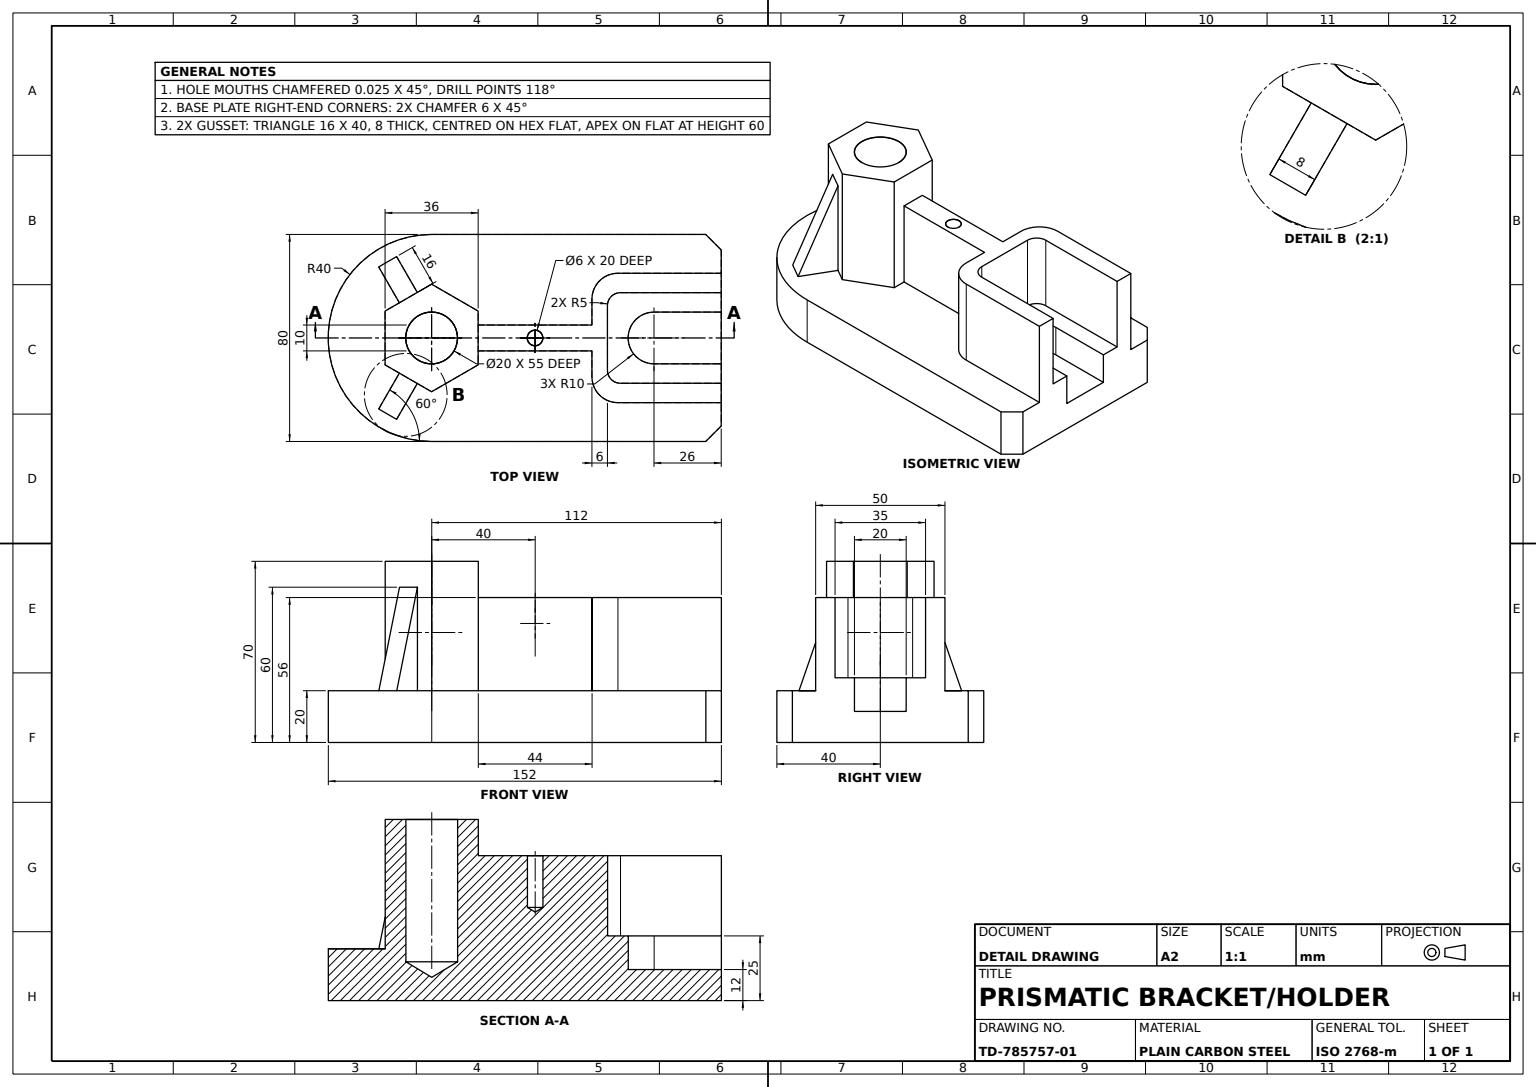
ISO-10303-21;
HEADER;
FILE_DESCRIPTION((''),'2;1');
FILE_NAME('','',(''),(''),'','','');
FILE_SCHEMA(('AUTOMOTIVE_DESIGN'));
ENDSEC;
DATA;
#1=APPLICATION_CONTEXT('');
#2=PRODUCT_CONTEXT('',#1,'mechanical');
#3=PRODUCT('','','',(#2));
#4=PRODUCT_DEFINITION_FORMATION('','',#3);
#5=PRODUCT_DEFINITION_CONTEXT('',#1,'design');
#6=PRODUCT_DEFINITION('','',#4,#5);
#7=PRODUCT_DEFINITION_SHAPE('','',#6);
#8=(LENGTH_UNIT()NAMED_UNIT(*)SI_UNIT(.MILLI.,.METRE.));
#9=(NAMED_UNIT(*)PLANE_ANGLE_UNIT()SI_UNIT($,.RADIAN.));
#10=(NAMED_UNIT(*)SI_UNIT($,.STERADIAN.)SOLID_ANGLE_UNIT());
#11=UNCERTAINTY_MEASURE_WITH_UNIT(LENGTH_MEASURE(1.E-05),#8,'distance_accuracy_value','');
#12=(GEOMETRIC_REPRESENTATION_CONTEXT(3)GLOBAL_UNCERTAINTY_ASSIGNED_CONTEXT((#11))GLOBAL_UNIT_ASSIGNED_CONTEXT((#8,#9,#10))REPRESENTATION_CONTEXT('',''));
#13=CARTESIAN_POINT('',(40.,36.,-3.));
#14=VERTEX_POINT('',#13);
#15=CARTESIAN_POINT('',(40.,55.975,-3.));
#16=VERTEX_POINT('',#15);
#17=CARTESIAN_POINT('',(40.,56.,-3.));
#18=DIRECTION('',(0.,1.,0.));
#19=VECTOR('',#18,1000.);
#20=LINE('',#17,#19);
#21=EDGE_CURVE('',#14,#16,#20,.T.);
#22=ORIENTED_EDGE('',*,*,#21,.T.);
#23=CARTESIAN_POINT('',(40.,55.975,3.));
#24=VERTEX_POINT('',#23);
#25=CARTESIAN_POINT('',(40.,55.975,0.));
#26=DIRECTION('',(0.,0.,1.));
#27=AXIS2_PLACEMENT_3D('',#25,#18,#26);
#28=CIRCLE('',#27,3.);
#29=EDGE_CURVE('',#16,#24,#28,.T.);
#30=ORIENTED_EDGE('',*,*,#29,.T.);
#31=CARTESIAN_POINT('',(40.,36.,3.));
#32=VERTEX_POINT('',#31);
#33=CARTESIAN_POINT('',(40.,56.,3.));
#34=LINE('',#33,#19);
#35=EDGE_CURVE('',#32,#24,#34,.T.);
#36=ORIENTED_EDGE('',*,*,#35,.F.);
#37=CARTESIAN_POINT('',(40.,36.,0.));
#38=AXIS2_PLACEMENT_3D('',#37,#18,#26);
#39=CIRCLE('',#38,3.);
#40=EDGE_CURVE('',#14,#32,#39,.T.);
#41=ORIENTED_EDGE('',*,*,#40,.F.);
#42=EDGE_LOOP('',(#22,#30,#36,#41));
#43=FACE_OUTER_BOUND('',#42,.T.);
#44=CARTESIAN_POINT('',(40.,56.,0.));
#45=AXIS2_PLACEMENT_3D('',#44,#18,#26);
#46=CYLINDRICAL_SURFACE('',#45,3.);
#47=ADVANCED_FACE('',(#43),#46,.F.);
#48=CARTESIAN_POINT('',(62.,56.,15.));
#49=VERTEX_POINT('',#48);
#50=CARTESIAN_POINT('',(62.,20.,15.));
#51=VERTEX_POINT('',#50);
#52=DIRECTION('',(0.,-1.,0.));
#53=VECTOR('',#52,1000.);
#54=LINE('',#48,#53);
#55=EDGE_CURVE('',#49,#51,#54,.T.);
#56=ORIENTED_EDGE('',*,*,#55,.F.);
#57=CARTESIAN_POINT('',(62.,56.,5.));
#58=VERTEX_POINT('',#57);
#59=VECTOR('',#26,1000.);
#60=LINE('',#57,#59);
#61=EDGE_CURVE('',#58,#49,#60,.T.);
#62=ORIENTED_EDGE('',*,*,#61,.F.);
#63=CARTESIAN_POINT('',(62.,20.,5.));
#64=VERTEX_POINT('',#63);
#65=LINE('',#57,#53);
#66=EDGE_CURVE('',#58,#64,#65,.T.);
#67=ORIENTED_EDGE('',*,*,#66,.T.);
#68=LINE('',#63,#59);
#69=EDGE_CURVE('',#64,#51,#68,.T.);
#70=ORIENTED_EDGE('',*,*,#69,.T.);
#71=EDGE_LOOP('',(#56,#62,#67,#70));
#72=FACE_OUTER_BOUND('',#71,.T.);
#73=DIRECTION('',(1.,0.,0.));
#74=DIRECTION('',(0.,0.,-1.));
#75=AXIS2_PLACEMENT_3D('',#57,#73,#74);
#76=PLANE('',#75);
#77=ADVANCED_FACE('',(#72),#76,.F.);
#78=CARTESIAN_POINT('',(68.,56.,12.5));
#79=VERTEX_POINT('',#78);
#80=CARTESIAN_POINT('',(68.,25.,12.5));
#81=VERTEX_POINT('',#80);
#82=LINE('',#78,#53);
#83=EDGE_CURVE('',#79,#81,#82,.T.);
#84=ORIENTED_EDGE('',*,*,#83,.F.);
#85=CARTESIAN_POINT('',(73.,56.,17.5));
#86=VERTEX_POINT('',#85);
#87=CARTESIAN_POINT('',(73.,56.,12.5));
#88=AXIS2_PLACEMENT_3D('',#87,#52,#74);
#89=CIRCLE('',#88,5.);
#90=EDGE_CURVE('',#86,#79,#89,.T.);
#91=ORIENTED_EDGE('',*,*,#90,.F.);
#92=CARTESIAN_POINT('',(73.,25.,17.5));
#93=VERTEX_POINT('',#92);
#94=LINE('',#85,#53);
#95=EDGE_CURVE('',#86,#93,#94,.T.);
#96=ORIENTED_EDGE('',*,*,#95,.T.);
#97=CARTESIAN_POINT('',(73.,25.,12.5));
#98=AXIS2_PLACEMENT_3D('',#97,#18,#26);
#99=CIRCLE('',#98,5.);
#100=EDGE_CURVE('',#81,#93,#99,.T.);
#101=ORIENTED_EDGE('',*,*,#100,.F.);
#102=EDGE_LOOP('',(#84,#91,#96,#101));
#103=FACE_OUTER_BOUND('',#102,.T.);
#104=CYLINDRICAL_SURFACE('',#88,5.);
#105=ADVANCED_FACE('',(#103),#104,.F.);
#106=CARTESIAN_POINT('',(68.,25.,-12.5));
#107=VERTEX_POINT('',#106);
#108=LINE('',#106,#59);
#109=EDGE_CURVE('',#107,#81,#108,.T.);
#110=ORIENTED_EDGE('',*,*,#109,.F.);
#111=CARTESIAN_POINT('',(68.,56.,-12.5));
#112=VERTEX_POINT('',#111);
#113=LINE('',#111,#53);
#114=EDGE_CURVE('',#112,#107,#113,.T.);
#115=ORIENTED_EDGE('',*,*,#114,.F.);
#116=VECTOR('',#74,1000.);
#117=LINE('',#78,#116);
#118=EDGE_CURVE('',#79,#112,#117,.T.);
#119=ORIENTED_EDGE('',*,*,#118,.F.);
#120=ORIENTED_EDGE('',*,*,#83,.T.);
#121=EDGE_LOOP('',(#110,#115,#119,#120));
#122=FACE_OUTER_BOUND('',#121,.T.);
#123=DIRECTION('',(-1.,0.,0.));
#124=AXIS2_PLACEMENT_3D('',#78,#123,#26);
#125=PLANE('',#124);
#126=ADVANCED_FACE('',(#122),#125,.F.);
#127=CARTESIAN_POINT('',(-12.464102,60.,-13.588457));
#128=VERTEX_POINT('',#127);
#129=CARTESIAN_POINT('',(-5.535898,60.,-17.588457));
#130=VERTEX_POINT('',#129);
#131=DIRECTION('',(0.866025404,0.,-0.5));
#132=VECTOR('',#131,1000.);
#133=LINE('',#129,#132);
#134=EDGE_CURVE('',#128,#130,#133,.T.);
#135=ORIENTED_EDGE('',*,*,#134,.T.);
#136=CARTESIAN_POINT('',(-13.535898,20.,-31.444864));
#137=VERTEX_POINT('',#136);
#138=CARTESIAN_POINT('',(-6.639347,54.482759,-19.499686));
#139=DIRECTION('',(0.185695338,0.928476691,0.32163376));
#140=VECTOR('',#139,1000.);
#141=LINE('',#138,#140);
#142=EDGE_CURVE('',#137,#130,#141,.T.);
#143=ORIENTED_EDGE('',*,*,#142,.F.);
#144=CARTESIAN_POINT('',(-20.464102,20.,-27.444864));
#145=VERTEX_POINT('',#144);
#146=DIRECTION('',(-0.866025404,0.,0.5));
#147=VECTOR('',#146,1000.);
#148=LINE('',#136,#147);
#149=EDGE_CURVE('',#137,#145,#148,.T.);
#150=ORIENTED_EDGE('',*,*,#149,.T.);
#151=LINE('',#127,#140);
#152=EDGE_CURVE('',#145,#128,#151,.T.);
#153=ORIENTED_EDGE('',*,*,#152,.T.);
#154=EDGE_LOOP('',(#135,#143,#150,#153));
#155=FACE_OUTER_BOUND('',#154,.T.);
#156=CARTESIAN_POINT('',(-221.915759,60.,107.338513));
#157=DIRECTION('',(0.464238345,-0.371390676,0.804084401));
#158=AXIS2_PLACEMENT_3D('',#156,#157,#131);
#159=PLANE('',#158);
#160=ADVANCED_FACE('',(#155),#159,.F.);
#161=CARTESIAN_POINT('',(106.,20.,-40.));
#162=VERTEX_POINT('',#161);
#163=CARTESIAN_POINT('',(106.,0.,-40.));
#164=VERTEX_POINT('',#163);
#165=LINE('',#161,#53);
#166=EDGE_CURVE('',#162,#164,#165,.T.);
#167=ORIENTED_EDGE('',*,*,#166,.F.);
#168=CARTESIAN_POINT('',(112.,20.,-34.));
#169=VERTEX_POINT('',#168);
#170=DIRECTION('',(-0.707106781,0.,-0.707106781));
#171=VECTOR('',#170,1000.);
#172=LINE('',#161,#171);
#173=EDGE_CURVE('',#169,#162,#172,.T.);
#174=ORIENTED_EDGE('',*,*,#173,.F.);
#175=CARTESIAN_POINT('',(112.,0.,-34.));
#176=VERTEX_POINT('',#175);
#177=LINE('',#168,#53);
#178=EDGE_CURVE('',#169,#176,#177,.T.);
#179=ORIENTED_EDGE('',*,*,#178,.T.);
#180=LINE('',#163,#171);
#181=EDGE_CURVE('',#176,#164,#180,.T.);
#182=ORIENTED_EDGE('',*,*,#181,.T.);
#183=EDGE_LOOP('',(#167,#174,#179,#182));
#184=FACE_OUTER_BOUND('',#183,.T.);
#185=DIRECTION('',(-0.707106781,0.,0.707106781));
#186=DIRECTION('',(0.707106781,0.,0.707106781));
#187=AXIS2_PLACEMENT_3D('',#161,#185,#186);
#188=PLANE('',#187);
#189=ADVANCED_FACE('',(#184),#188,.F.);
#190=CARTESIAN_POINT('',(-13.535898,20.,31.444864));
#191=VERTEX_POINT('',#190);
#192=CARTESIAN_POINT('',(-5.535898,20.,17.588457));
#193=VERTEX_POINT('',#192);
#194=DIRECTION('',(0.5,0.,-0.866025404));
#195=VECTOR('',#194,1000.);
#196=LINE('',#190,#195);
#197=EDGE_CURVE('',#191,#193,#196,.T.);
#198=ORIENTED_EDGE('',*,*,#197,.F.);
#199=CARTESIAN_POINT('',(-20.464102,20.,27.444864));
#200=VERTEX_POINT('',#199);
#201=DIRECTION('',(0.866025404,0.,0.5));
#202=VECTOR('',#201,1000.);
#203=LINE('',#199,#202);
#204=EDGE_CURVE('',#200,#191,#203,.T.);
#205=ORIENTED_EDGE('',*,*,#204,.F.);
#206=CARTESIAN_POINT('',(-12.464102,20.,13.588457));
#207=VERTEX_POINT('',#206);
#208=LINE('',#199,#195);
#209=EDGE_CURVE('',#200,#207,#208,.T.);
#210=ORIENTED_EDGE('',*,*,#209,.T.);
#211=CARTESIAN_POINT('',(-18.,20.,10.392305));
#212=VERTEX_POINT('',#211);
#213=LINE('',#211,#202);
#214=EDGE_CURVE('',#212,#207,#213,.T.);
#215=ORIENTED_EDGE('',*,*,#214,.F.);
#216=CARTESIAN_POINT('',(-18.,20.,-10.392305));
#217=VERTEX_POINT('',#216);
#218=LINE('',#216,#59);
#219=EDGE_CURVE('',#217,#212,#218,.T.);
#220=ORIENTED_EDGE('',*,*,#219,.F.);
#221=CARTESIAN_POINT('',(-12.464102,20.,-13.588457));
#222=VERTEX_POINT('',#221);
#223=CARTESIAN_POINT('',(0.,20.,-20.78461));
#224=LINE('',#223,#147);
#225=EDGE_CURVE('',#222,#217,#224,.T.);
#226=ORIENTED_EDGE('',*,*,#225,.F.);
#227=DIRECTION('',(0.5,0.,0.866025404));
#228=VECTOR('',#227,1000.);
#229=LINE('',#144,#228);
#230=EDGE_CURVE('',#145,#222,#229,.T.);
#231=ORIENTED_EDGE('',*,*,#230,.F.);
#232=ORIENTED_EDGE('',*,*,#149,.F.);
#233=CARTESIAN_POINT('',(-5.535898,20.,-17.588457));
#234=VERTEX_POINT('',#233);
#235=LINE('',#136,#228);
#236=EDGE_CURVE('',#137,#234,#235,.T.);
#237=ORIENTED_EDGE('',*,*,#236,.T.);
#238=VERTEX_POINT('',#223);
#239=EDGE_CURVE('',#238,#234,#224,.T.);
#240=ORIENTED_EDGE('',*,*,#239,.F.);
#241=CARTESIAN_POINT('',(18.,20.,-10.392305));
#242=VERTEX_POINT('',#241);
#243=DIRECTION('',(-0.866025404,0.,-0.5));
#244=VECTOR('',#243,1000.);
#245=LINE('',#241,#244);
#246=EDGE_CURVE('',#242,#238,#245,.T.);
#247=ORIENTED_EDGE('',*,*,#246,.F.);
#248=CARTESIAN_POINT('',(18.,20.,-5.));
#249=VERTEX_POINT('',#248);
#250=CARTESIAN_POINT('',(18.,20.,10.392305));
#251=LINE('',#250,#116);
#252=EDGE_CURVE('',#249,#242,#251,.T.);
#253=ORIENTED_EDGE('',*,*,#252,.F.);
#254=CARTESIAN_POINT('',(62.,20.,-5.));
#255=VERTEX_POINT('',#254);
#256=VECTOR('',#123,1000.);
#257=LINE('',#248,#256);
#258=EDGE_CURVE('',#255,#249,#257,.T.);
#259=ORIENTED_EDGE('',*,*,#258,.F.);
#260=CARTESIAN_POINT('',(62.,20.,-15.));
#261=VERTEX_POINT('',#260);
#262=LINE('',#260,#59);
#263=EDGE_CURVE('',#261,#255,#262,.T.);
#264=ORIENTED_EDGE('',*,*,#263,.F.);
#265=CARTESIAN_POINT('',(72.,20.,-25.));
#266=VERTEX_POINT('',#265);
#267=CARTESIAN_POINT('',(72.,20.,-15.));
#268=AXIS2_PLACEMENT_3D('',#267,#18,#26);
#269=CIRCLE('',#268,10.);
#270=EDGE_CURVE('',#266,#261,#269,.T.);
#271=ORIENTED_EDGE('',*,*,#270,.F.);
#272=CARTESIAN_POINT('',(112.,20.,-25.));
#273=VERTEX_POINT('',#272);
#274=LINE('',#272,#256);
#275=EDGE_CURVE('',#273,#266,#274,.T.);
#276=ORIENTED_EDGE('',*,*,#275,.F.);
#277=LINE('',#168,#116);
#278=EDGE_CURVE('',#273,#169,#277,.T.);
#279=ORIENTED_EDGE('',*,*,#278,.T.);
#280=ORIENTED_EDGE('',*,*,#173,.T.);
#281=CARTESIAN_POINT('',(0.,20.,-40.));
#282=VERTEX_POINT('',#281);
#283=LINE('',#281,#256);
#284=EDGE_CURVE('',#162,#282,#283,.T.);
#285=ORIENTED_EDGE('',*,*,#284,.T.);
#286=CARTESIAN_POINT('',(0.,20.,40.));
#287=VERTEX_POINT('',#286);
#288=CARTESIAN_POINT('',(0.,20.,0.));
#289=AXIS2_PLACEMENT_3D('',#288,#18,#26);
#290=CIRCLE('',#289,40.);
#291=EDGE_CURVE('',#282,#287,#290,.T.);
#292=ORIENTED_EDGE('',*,*,#291,.T.);
#293=CARTESIAN_POINT('',(106.,20.,40.));
#294=VERTEX_POINT('',#293);
#295=VECTOR('',#73,1000.);
#296=LINE('',#293,#295);
#297=EDGE_CURVE('',#287,#294,#296,.T.);
#298=ORIENTED_EDGE('',*,*,#297,.T.);
#299=CARTESIAN_POINT('',(112.,20.,34.));
#300=VERTEX_POINT('',#299);
#301=DIRECTION('',(0.707106781,0.,-0.707106781));
#302=VECTOR('',#301,1000.);
#303=LINE('',#299,#302);
#304=EDGE_CURVE('',#294,#300,#303,.T.);
#305=ORIENTED_EDGE('',*,*,#304,.T.);
#306=CARTESIAN_POINT('',(112.,20.,25.));
#307=VERTEX_POINT('',#306);
#308=EDGE_CURVE('',#300,#307,#277,.T.);
#309=ORIENTED_EDGE('',*,*,#308,.T.);
#310=CARTESIAN_POINT('',(72.,20.,25.));
#311=VERTEX_POINT('',#310);
#312=LINE('',#310,#295);
#313=EDGE_CURVE('',#311,#307,#312,.T.);
#314=ORIENTED_EDGE('',*,*,#313,.F.);
#315=CARTESIAN_POINT('',(72.,20.,15.));
#316=AXIS2_PLACEMENT_3D('',#315,#18,#26);
#317=CIRCLE('',#316,10.);
#318=EDGE_CURVE('',#51,#311,#317,.T.);
#319=ORIENTED_EDGE('',*,*,#318,.F.);
#320=ORIENTED_EDGE('',*,*,#69,.F.);
#321=CARTESIAN_POINT('',(18.,20.,5.));
#322=VERTEX_POINT('',#321);
#323=LINE('',#321,#295);
#324=EDGE_CURVE('',#322,#64,#323,.T.);
#325=ORIENTED_EDGE('',*,*,#324,.F.);
#326=VERTEX_POINT('',#250);
#327=EDGE_CURVE('',#326,#322,#251,.T.);
#328=ORIENTED_EDGE('',*,*,#327,.F.);
#329=CARTESIAN_POINT('',(0.,20.,20.78461));
#330=VERTEX_POINT('',#329);
#331=LINE('',#329,#132);
#332=EDGE_CURVE('',#330,#326,#331,.T.);
#333=ORIENTED_EDGE('',*,*,#332,.F.);
#334=EDGE_CURVE('',#193,#330,#213,.T.);
#335=ORIENTED_EDGE('',*,*,#334,.F.);
#336=EDGE_LOOP('',(#198,#205,#210,#215,#220,#226,#231,#232,#237,#240,#247,#253,#259,#264,#271,#276,#279,#280,#285,#292,#298,#305,#309,#314,#319,#320,#325,#328,#333,#335));
#337=FACE_OUTER_BOUND('',#336,.T.);
#338=PLANE('',#289);
#339=ADVANCED_FACE('',(#337),#338,.T.);
#340=CARTESIAN_POINT('',(112.,25.,10.));
#341=VERTEX_POINT('',#340);
#342=CARTESIAN_POINT('',(86.,25.,10.));
#343=VERTEX_POINT('',#342);
#344=LINE('',#340,#256);
#345=EDGE_CURVE('',#341,#343,#344,.T.);
#346=ORIENTED_EDGE('',*,*,#345,.T.);
#347=CARTESIAN_POINT('',(86.,25.,-10.));
#348=VERTEX_POINT('',#347);
#349=CARTESIAN_POINT('',(86.,25.,0.));
#350=AXIS2_PLACEMENT_3D('',#349,#52,#74);
#351=CIRCLE('',#350,10.);
#352=EDGE_CURVE('',#343,#348,#351,.T.);
#353=ORIENTED_EDGE('',*,*,#352,.T.);
#354=CARTESIAN_POINT('',(112.,25.,-10.));
#355=VERTEX_POINT('',#354);
#356=LINE('',#347,#295);
#357=EDGE_CURVE('',#348,#355,#356,.T.);
#358=ORIENTED_EDGE('',*,*,#357,.T.);
#359=CARTESIAN_POINT('',(112.,25.,-17.5));
#360=VERTEX_POINT('',#359);
#361=LINE('',#354,#116);
#362=EDGE_CURVE('',#355,#360,#361,.T.);
#363=ORIENTED_EDGE('',*,*,#362,.T.);
#364=CARTESIAN_POINT('',(73.,25.,-17.5));
#365=VERTEX_POINT('',#364);
#366=LINE('',#359,#256);
#367=EDGE_CURVE('',#360,#365,#366,.T.);
#368=ORIENTED_EDGE('',*,*,#367,.T.);
#369=CARTESIAN_POINT('',(73.,25.,-12.5));
#370=AXIS2_PLACEMENT_3D('',#369,#18,#26);
#371=CIRCLE('',#370,5.);
#372=EDGE_CURVE('',#365,#107,#371,.T.);
#373=ORIENTED_EDGE('',*,*,#372,.T.);
#374=ORIENTED_EDGE('',*,*,#109,.T.);
#375=ORIENTED_EDGE('',*,*,#100,.T.);
#376=CARTESIAN_POINT('',(112.,25.,17.5));
#377=VERTEX_POINT('',#376);
#378=LINE('',#92,#295);
#379=EDGE_CURVE('',#93,#377,#378,.T.);
#380=ORIENTED_EDGE('',*,*,#379,.T.);
#381=LINE('',#376,#116);
#382=EDGE_CURVE('',#377,#341,#381,.T.);
#383=ORIENTED_EDGE('',*,*,#382,.T.);
#384=EDGE_LOOP('',(#346,#353,#358,#363,#368,#373,#374,#375,#380,#383));
#385=FACE_OUTER_BOUND('',#384,.T.);
#386=PLANE('',#370);
#387=ADVANCED_FACE('',(#385),#386,.T.);
#388=ORIENTED_EDGE('',*,*,#313,.T.);
#389=CARTESIAN_POINT('',(112.,56.,25.));
#390=VERTEX_POINT('',#389);
#391=LINE('',#389,#53);
#392=EDGE_CURVE('',#390,#307,#391,.T.);
#393=ORIENTED_EDGE('',*,*,#392,.F.);
#394=CARTESIAN_POINT('',(72.,56.,25.));
#395=VERTEX_POINT('',#394);
#396=LINE('',#394,#295);
#397=EDGE_CURVE('',#395,#390,#396,.T.);
#398=ORIENTED_EDGE('',*,*,#397,.F.);
#399=LINE('',#394,#53);
#400=EDGE_CURVE('',#395,#311,#399,.T.);
#401=ORIENTED_EDGE('',*,*,#400,.T.);
#402=EDGE_LOOP('',(#388,#393,#398,#401));
#403=FACE_OUTER_BOUND('',#402,.T.);
#404=AXIS2_PLACEMENT_3D('',#394,#74,#123);
#405=PLANE('',#404);
#406=ADVANCED_FACE('',(#403),#405,.F.);
#407=EDGE_CURVE('',#24,#16,#28,.T.);
#408=ORIENTED_EDGE('',*,*,#407,.F.);
#409=CARTESIAN_POINT('',(40.,56.,3.025));
#410=VERTEX_POINT('',#409);
#411=DIRECTION('',(0.,0.707106781,0.707106781));
#412=VECTOR('',#411,1000.);
#413=LINE('',#409,#412);
#414=EDGE_CURVE('',#24,#410,#413,.T.);
#415=ORIENTED_EDGE('',*,*,#414,.T.);
#416=CARTESIAN_POINT('',(40.,56.,-3.025));
#417=VERTEX_POINT('',#416);
#418=CIRCLE('',#45,3.025);
#419=EDGE_CURVE('',#410,#417,#418,.T.);
#420=ORIENTED_EDGE('',*,*,#419,.T.);
#421=DIRECTION('',(0.,0.707106781,-0.707106781));
#422=VECTOR('',#421,1000.);
#423=LINE('',#416,#422);
#424=EDGE_CURVE('',#16,#417,#423,.T.);
#425=ORIENTED_EDGE('',*,*,#424,.F.);
#426=EDGE_LOOP('',(#408,#415,#420,#425));
#427=FACE_OUTER_BOUND('',#426,.T.);
#428=CONICAL_SURFACE('',#45,3.025,0.785398163);
#429=ADVANCED_FACE('',(#427),#428,.F.);
#430=CARTESIAN_POINT('',(0.,0.,-40.));
#431=VERTEX_POINT('',#430);
#432=LINE('',#430,#256);
#433=EDGE_CURVE('',#164,#431,#432,.T.);
#434=ORIENTED_EDGE('',*,*,#433,.T.);
#435=LINE('',#281,#53);
#436=EDGE_CURVE('',#282,#431,#435,.T.);
#437=ORIENTED_EDGE('',*,*,#436,.F.);
#438=ORIENTED_EDGE('',*,*,#284,.F.);
#439=ORIENTED_EDGE('',*,*,#166,.T.);
#440=EDGE_LOOP('',(#434,#437,#438,#439));
#441=FACE_OUTER_BOUND('',#440,.T.);
#442=AXIS2_PLACEMENT_3D('',#281,#26,#73);
#443=PLANE('',#442);
#444=ADVANCED_FACE('',(#441),#443,.F.);
#445=CARTESIAN_POINT('',(0.,8.991394,0.));
#446=VERTEX_POINT('',#445);
#447=CARTESIAN_POINT('',(0.,15.,10.));
#448=VERTEX_POINT('',#447);
#449=DIRECTION('',(0.,0.515038075,0.857167301));
#450=VECTOR('',#449,1000.);
#451=LINE('',#447,#450);
#452=EDGE_CURVE('',#446,#448,#451,.T.);
#453=ORIENTED_EDGE('',*,*,#452,.T.);
#454=CARTESIAN_POINT('',(0.,15.,-10.));
#455=VERTEX_POINT('',#454);
#456=CARTESIAN_POINT('',(0.,15.,0.));
#457=AXIS2_PLACEMENT_3D('',#456,#18,#26);
#458=CIRCLE('',#457,10.);
#459=EDGE_CURVE('',#448,#455,#458,.T.);
#460=ORIENTED_EDGE('',*,*,#459,.T.);
#461=DIRECTION('',(0.,0.515038075,-0.857167301));
#462=VECTOR('',#461,1000.);
#463=LINE('',#454,#462);
#464=EDGE_CURVE('',#446,#455,#463,.T.);
#465=ORIENTED_EDGE('',*,*,#464,.F.);
#466=EDGE_LOOP('',(#453,#460,#465));
#467=FACE_OUTER_BOUND('',#466,.T.);
#468=CONICAL_SURFACE('',#457,10.,1.029744259);
#469=ADVANCED_FACE('',(#467),#468,.F.);
#470=CARTESIAN_POINT('',(106.,0.,40.));
#471=VERTEX_POINT('',#470);
#472=CARTESIAN_POINT('',(112.,0.,34.));
#473=VERTEX_POINT('',#472);
#474=LINE('',#472,#302);
#475=EDGE_CURVE('',#471,#473,#474,.T.);
#476=ORIENTED_EDGE('',*,*,#475,.T.);
#477=LINE('',#299,#53);
#478=EDGE_CURVE('',#300,#473,#477,.T.);
#479=ORIENTED_EDGE('',*,*,#478,.F.);
#480=ORIENTED_EDGE('',*,*,#304,.F.);
#481=LINE('',#293,#53);
#482=EDGE_CURVE('',#294,#471,#481,.T.);
#483=ORIENTED_EDGE('',*,*,#482,.T.);
#484=EDGE_LOOP('',(#476,#479,#480,#483));
#485=FACE_OUTER_BOUND('',#484,.T.);
#486=AXIS2_PLACEMENT_3D('',#299,#170,#185);
#487=PLANE('',#486);
#488=ADVANCED_FACE('',(#485),#487,.F.);
#489=CARTESIAN_POINT('',(0.,69.975,10.));
#490=VERTEX_POINT('',#489);
#491=CARTESIAN_POINT('',(0.,70.,10.025));
#492=VERTEX_POINT('',#491);
#493=LINE('',#491,#412);
#494=EDGE_CURVE('',#490,#492,#493,.T.);
#495=ORIENTED_EDGE('',*,*,#494,.T.);
#496=CARTESIAN_POINT('',(0.,70.,-10.025));
#497=VERTEX_POINT('',#496);
#498=CARTESIAN_POINT('',(0.,70.,0.));
#499=AXIS2_PLACEMENT_3D('',#498,#18,#26);
#500=CIRCLE('',#499,10.025);
#501=EDGE_CURVE('',#492,#497,#500,.T.);
#502=ORIENTED_EDGE('',*,*,#501,.T.);
#503=CARTESIAN_POINT('',(0.,69.975,-10.));
#504=VERTEX_POINT('',#503);
#505=LINE('',#496,#422);
#506=EDGE_CURVE('',#504,#497,#505,.T.);
#507=ORIENTED_EDGE('',*,*,#506,.F.);
#508=CARTESIAN_POINT('',(0.,69.975,0.));
#509=AXIS2_PLACEMENT_3D('',#508,#18,#26);
#510=CIRCLE('',#509,10.);
#511=EDGE_CURVE('',#490,#504,#510,.T.);
#512=ORIENTED_EDGE('',*,*,#511,.F.);
#513=EDGE_LOOP('',(#495,#502,#507,#512));
#514=FACE_OUTER_BOUND('',#513,.T.);
#515=CONICAL_SURFACE('',#499,10.025,0.785398163);
#516=ADVANCED_FACE('',(#514),#515,.F.);
#517=ORIENTED_EDGE('',*,*,#414,.F.);
#518=ORIENTED_EDGE('',*,*,#29,.F.);
#519=ORIENTED_EDGE('',*,*,#424,.T.);
#520=EDGE_CURVE('',#417,#410,#418,.T.);
#521=ORIENTED_EDGE('',*,*,#520,.T.);
#522=EDGE_LOOP('',(#517,#518,#519,#521));
#523=FACE_OUTER_BOUND('',#522,.T.);
#524=ADVANCED_FACE('',(#523),#428,.F.);
#525=ORIENTED_EDGE('',*,*,#452,.F.);
#526=ORIENTED_EDGE('',*,*,#464,.T.);
#527=EDGE_CURVE('',#455,#448,#458,.T.);
#528=ORIENTED_EDGE('',*,*,#527,.T.);
#529=EDGE_LOOP('',(#525,#526,#528));
#530=FACE_OUTER_BOUND('',#529,.T.);
#531=ADVANCED_FACE('',(#530),#468,.F.);
#532=ORIENTED_EDGE('',*,*,#197,.T.);
#533=CARTESIAN_POINT('',(-5.535898,60.,17.588457));
#534=VERTEX_POINT('',#533);
#535=LINE('',#533,#19);
#536=EDGE_CURVE('',#193,#534,#535,.T.);
#537=ORIENTED_EDGE('',*,*,#536,.T.);
#538=DIRECTION('',(0.185695338,0.928476691,-0.32163376));
#539=VECTOR('',#538,1000.);
#540=LINE('',#533,#539);
#541=EDGE_CURVE('',#191,#534,#540,.T.);
#542=ORIENTED_EDGE('',*,*,#541,.F.);
#543=EDGE_LOOP('',(#532,#537,#542));
#544=FACE_OUTER_BOUND('',#543,.T.);
#545=CARTESIAN_POINT('',(-13.535898,60.,31.444864));
#546=DIRECTION('',(-0.5,0.,0.866025404));
#547=AXIS2_PLACEMENT_3D('',#545,#243,#546);
#548=PLANE('',#547);
#549=ADVANCED_FACE('',(#544),#548,.F.);
#550=ORIENTED_EDGE('',*,*,#152,.F.);
#551=ORIENTED_EDGE('',*,*,#230,.T.);
#552=LINE('',#127,#19);
#553=EDGE_CURVE('',#222,#128,#552,.T.);
#554=ORIENTED_EDGE('',*,*,#553,.T.);
#555=EDGE_LOOP('',(#550,#551,#554));
#556=FACE_OUTER_BOUND('',#555,.T.);
#557=CARTESIAN_POINT('',(-20.464102,60.,-27.444864));
#558=DIRECTION('',(-0.5,0.,-0.866025404));
#559=AXIS2_PLACEMENT_3D('',#557,#131,#558);
#560=PLANE('',#559);
#561=ADVANCED_FACE('',(#556),#560,.F.);
#562=ORIENTED_EDGE('',*,*,#291,.F.);
#563=ORIENTED_EDGE('',*,*,#436,.T.);
#564=CARTESIAN_POINT('',(0.,0.,40.));
#565=VERTEX_POINT('',#564);
#566=CARTESIAN_POINT('',(0.,0.,0.));
#567=AXIS2_PLACEMENT_3D('',#566,#18,#26);
#568=CIRCLE('',#567,40.);
#569=EDGE_CURVE('',#431,#565,#568,.T.);
#570=ORIENTED_EDGE('',*,*,#569,.T.);
#571=LINE('',#286,#53);
#572=EDGE_CURVE('',#287,#565,#571,.T.);
#573=ORIENTED_EDGE('',*,*,#572,.F.);
#574=EDGE_LOOP('',(#562,#563,#570,#573));
#575=FACE_OUTER_BOUND('',#574,.T.);
#576=AXIS2_PLACEMENT_3D('',#288,#52,#74);
#577=CYLINDRICAL_SURFACE('',#576,40.);
#578=ADVANCED_FACE('',(#575),#577,.T.);
#579=CARTESIAN_POINT('',(112.,56.,-25.));
#580=VERTEX_POINT('',#579);
#581=CARTESIAN_POINT('',(72.,56.,-25.));
#582=VERTEX_POINT('',#581);
#583=LINE('',#579,#256);
#584=EDGE_CURVE('',#580,#582,#583,.T.);
#585=ORIENTED_EDGE('',*,*,#584,.F.);
#586=LINE('',#579,#53);
#587=EDGE_CURVE('',#580,#273,#586,.T.);
#588=ORIENTED_EDGE('',*,*,#587,.T.);
#589=ORIENTED_EDGE('',*,*,#275,.T.);
#590=LINE('',#581,#53);
#591=EDGE_CURVE('',#582,#266,#590,.T.);
#592=ORIENTED_EDGE('',*,*,#591,.F.);
#593=EDGE_LOOP('',(#585,#588,#589,#592));
#594=FACE_OUTER_BOUND('',#593,.T.);
#595=AXIS2_PLACEMENT_3D('',#579,#26,#73);
#596=PLANE('',#595);
#597=ADVANCED_FACE('',(#594),#596,.F.);
#598=CARTESIAN_POINT('',(0.,70.,-10.));
#599=LINE('',#598,#19);
#600=EDGE_CURVE('',#455,#504,#599,.T.);
#601=ORIENTED_EDGE('',*,*,#600,.T.);
#602=EDGE_CURVE('',#504,#490,#510,.T.);
#603=ORIENTED_EDGE('',*,*,#602,.T.);
#604=CARTESIAN_POINT('',(0.,70.,10.));
#605=LINE('',#604,#19);
#606=EDGE_CURVE('',#448,#490,#605,.T.);
#607=ORIENTED_EDGE('',*,*,#606,.F.);
#608=ORIENTED_EDGE('',*,*,#527,.F.);
#609=EDGE_LOOP('',(#601,#603,#607,#608));
#610=FACE_OUTER_BOUND('',#609,.T.);
#611=CYLINDRICAL_SURFACE('',#499,10.);
#612=ADVANCED_FACE('',(#610),#611,.F.);
#613=CARTESIAN_POINT('',(18.,70.,-10.392305));
#614=VERTEX_POINT('',#613);
#615=CARTESIAN_POINT('',(0.,70.,-20.78461));
#616=VERTEX_POINT('',#615);
#617=LINE('',#613,#244);
#618=EDGE_CURVE('',#614,#616,#617,.T.);
#619=ORIENTED_EDGE('',*,*,#618,.T.);
#620=CARTESIAN_POINT('',(-18.,70.,-10.392305));
#621=VERTEX_POINT('',#620);
#622=LINE('',#615,#147);
#623=EDGE_CURVE('',#616,#621,#622,.T.);
#624=ORIENTED_EDGE('',*,*,#623,.T.);
#625=CARTESIAN_POINT('',(-18.,70.,10.392305));
#626=VERTEX_POINT('',#625);
#627=LINE('',#620,#59);
#628=EDGE_CURVE('',#621,#626,#627,.T.);
#629=ORIENTED_EDGE('',*,*,#628,.T.);
#630=CARTESIAN_POINT('',(0.,70.,20.78461));
#631=VERTEX_POINT('',#630);
#632=LINE('',#625,#202);
#633=EDGE_CURVE('',#626,#631,#632,.T.);
#634=ORIENTED_EDGE('',*,*,#633,.T.);
#635=CARTESIAN_POINT('',(18.,70.,10.392305));
#636=VERTEX_POINT('',#635);
#637=LINE('',#630,#132);
#638=EDGE_CURVE('',#631,#636,#637,.T.);
#639=ORIENTED_EDGE('',*,*,#638,.T.);
#640=LINE('',#635,#116);
#641=EDGE_CURVE('',#636,#614,#640,.T.);
#642=ORIENTED_EDGE('',*,*,#641,.T.);
#643=EDGE_LOOP('',(#619,#624,#629,#634,#639,#642));
#644=FACE_OUTER_BOUND('',#643,.T.);
#645=EDGE_CURVE('',#497,#492,#500,.T.);
#646=ORIENTED_EDGE('',*,*,#645,.F.);
#647=ORIENTED_EDGE('',*,*,#501,.F.);
#648=EDGE_LOOP('',(#646,#647));
#649=FACE_BOUND('',#648,.T.);
#650=PLANE('',#499);
#651=ADVANCED_FACE('',(#644,#649),#650,.T.);
#652=CARTESIAN_POINT('',(18.,56.,5.));
#653=VERTEX_POINT('',#652);
#654=LINE('',#652,#53);
#655=EDGE_CURVE('',#653,#322,#654,.T.);
#656=ORIENTED_EDGE('',*,*,#655,.F.);
#657=CARTESIAN_POINT('',(18.,56.,-5.));
#658=VERTEX_POINT('',#657);
#659=LINE('',#657,#59);
#660=EDGE_CURVE('',#658,#653,#659,.T.);
#661=ORIENTED_EDGE('',*,*,#660,.F.);
#662=LINE('',#657,#53);
#663=EDGE_CURVE('',#658,#249,#662,.T.);
#664=ORIENTED_EDGE('',*,*,#663,.T.);
#665=ORIENTED_EDGE('',*,*,#252,.T.);
#666=LINE('',#613,#53);
#667=EDGE_CURVE('',#614,#242,#666,.T.);
#668=ORIENTED_EDGE('',*,*,#667,.F.);
#669=ORIENTED_EDGE('',*,*,#641,.F.);
#670=LINE('',#635,#53);
#671=EDGE_CURVE('',#636,#326,#670,.T.);
#672=ORIENTED_EDGE('',*,*,#671,.T.);
#673=ORIENTED_EDGE('',*,*,#327,.T.);
#674=EDGE_LOOP('',(#656,#661,#664,#665,#668,#669,#672,#673));
#675=FACE_OUTER_BOUND('',#674,.T.);
#676=AXIS2_PLACEMENT_3D('',#635,#123,#26);
#677=PLANE('',#676);
#678=ADVANCED_FACE('',(#675),#677,.F.);
#679=ORIENTED_EDGE('',*,*,#591,.T.);
#680=ORIENTED_EDGE('',*,*,#270,.T.);
#681=CARTESIAN_POINT('',(62.,56.,-15.));
#682=VERTEX_POINT('',#681);
#683=LINE('',#681,#53);
#684=EDGE_CURVE('',#682,#261,#683,.T.);
#685=ORIENTED_EDGE('',*,*,#684,.F.);
#686=CARTESIAN_POINT('',(72.,56.,-15.));
#687=AXIS2_PLACEMENT_3D('',#686,#18,#26);
#688=CIRCLE('',#687,10.);
#689=EDGE_CURVE('',#582,#682,#688,.T.);
#690=ORIENTED_EDGE('',*,*,#689,.F.);
#691=EDGE_LOOP('',(#679,#680,#685,#690));
#692=FACE_OUTER_BOUND('',#691,.T.);
#693=AXIS2_PLACEMENT_3D('',#686,#52,#74);
#694=CYLINDRICAL_SURFACE('',#693,10.);
#695=ADVANCED_FACE('',(#692),#694,.T.);
#696=CARTESIAN_POINT('',(112.,12.,-10.));
#697=VERTEX_POINT('',#696);
#698=LINE('',#696,#19);
#699=EDGE_CURVE('',#697,#355,#698,.T.);
#700=ORIENTED_EDGE('',*,*,#699,.T.);
#701=ORIENTED_EDGE('',*,*,#357,.F.);
#702=CARTESIAN_POINT('',(86.,12.,-10.));
#703=VERTEX_POINT('',#702);
#704=LINE('',#702,#19);
#705=EDGE_CURVE('',#703,#348,#704,.T.);
#706=ORIENTED_EDGE('',*,*,#705,.F.);
#707=LINE('',#702,#256);
#708=EDGE_CURVE('',#697,#703,#707,.T.);
#709=ORIENTED_EDGE('',*,*,#708,.F.);
#710=EDGE_LOOP('',(#700,#701,#706,#709));
#711=FACE_OUTER_BOUND('',#710,.T.);
#712=AXIS2_PLACEMENT_3D('',#702,#74,#123);
#713=PLANE('',#712);
#714=ADVANCED_FACE('',(#711),#713,.F.);
#715=ORIENTED_EDGE('',*,*,#352,.F.);
#716=CARTESIAN_POINT('',(86.,12.,10.));
#717=VERTEX_POINT('',#716);
#718=LINE('',#716,#19);
#719=EDGE_CURVE('',#717,#343,#718,.T.);
#720=ORIENTED_EDGE('',*,*,#719,.F.);
#721=CARTESIAN_POINT('',(86.,12.,0.));
#722=AXIS2_PLACEMENT_3D('',#721,#18,#26);
#723=CIRCLE('',#722,10.);
#724=EDGE_CURVE('',#703,#717,#723,.T.);
#725=ORIENTED_EDGE('',*,*,#724,.F.);
#726=ORIENTED_EDGE('',*,*,#705,.T.);
#727=EDGE_LOOP('',(#715,#720,#725,#726));
#728=FACE_OUTER_BOUND('',#727,.T.);
#729=CYLINDRICAL_SURFACE('',#722,10.);
#730=ADVANCED_FACE('',(#728),#729,.F.);
#731=ORIENTED_EDGE('',*,*,#584,.T.);
#732=ORIENTED_EDGE('',*,*,#689,.T.);
#733=CARTESIAN_POINT('',(62.,56.,-5.));
#734=VERTEX_POINT('',#733);
#735=LINE('',#681,#59);
#736=EDGE_CURVE('',#682,#734,#735,.T.);
#737=ORIENTED_EDGE('',*,*,#736,.T.);
#738=LINE('',#657,#256);
#739=EDGE_CURVE('',#734,#658,#738,.T.);
#740=ORIENTED_EDGE('',*,*,#739,.T.);
#741=ORIENTED_EDGE('',*,*,#660,.T.);
#742=LINE('',#652,#295);
#743=EDGE_CURVE('',#653,#58,#742,.T.);
#744=ORIENTED_EDGE('',*,*,#743,.T.);
#745=ORIENTED_EDGE('',*,*,#61,.T.);
#746=CARTESIAN_POINT('',(72.,56.,15.));
#747=AXIS2_PLACEMENT_3D('',#746,#18,#26);
#748=CIRCLE('',#747,10.);
#749=EDGE_CURVE('',#49,#395,#748,.T.);
#750=ORIENTED_EDGE('',*,*,#749,.T.);
#751=ORIENTED_EDGE('',*,*,#397,.T.);
#752=CARTESIAN_POINT('',(112.,56.,17.5));
#753=VERTEX_POINT('',#752);
#754=LINE('',#389,#116);
#755=EDGE_CURVE('',#390,#753,#754,.T.);
#756=ORIENTED_EDGE('',*,*,#755,.T.);
#757=LINE('',#752,#256);
#758=EDGE_CURVE('',#753,#86,#757,.T.);
#759=ORIENTED_EDGE('',*,*,#758,.T.);
#760=ORIENTED_EDGE('',*,*,#90,.T.);
#761=ORIENTED_EDGE('',*,*,#118,.T.);
#762=CARTESIAN_POINT('',(73.,56.,-17.5));
#763=VERTEX_POINT('',#762);
#764=CARTESIAN_POINT('',(73.,56.,-12.5));
#765=AXIS2_PLACEMENT_3D('',#764,#52,#74);
#766=CIRCLE('',#765,5.);
#767=EDGE_CURVE('',#112,#763,#766,.T.);
#768=ORIENTED_EDGE('',*,*,#767,.T.);
#769=CARTESIAN_POINT('',(112.,56.,-17.5));
#770=VERTEX_POINT('',#769);
#771=LINE('',#762,#295);
#772=EDGE_CURVE('',#763,#770,#771,.T.);
#773=ORIENTED_EDGE('',*,*,#772,.T.);
#774=LINE('',#769,#116);
#775=EDGE_CURVE('',#770,#580,#774,.T.);
#776=ORIENTED_EDGE('',*,*,#775,.T.);
#777=EDGE_LOOP('',(#731,#732,#737,#740,#741,#744,#745,#750,#751,#756,#759,#760,#761,#768,#773,#776));
#778=FACE_OUTER_BOUND('',#777,.T.);
#779=ORIENTED_EDGE('',*,*,#520,.F.);
#780=ORIENTED_EDGE('',*,*,#419,.F.);
#781=EDGE_LOOP('',(#779,#780));
#782=FACE_BOUND('',#781,.T.);
#783=PLANE('',#747);
#784=ADVANCED_FACE('',(#778,#782),#783,.T.);
#785=ORIENTED_EDGE('',*,*,#749,.F.);
#786=ORIENTED_EDGE('',*,*,#55,.T.);
#787=ORIENTED_EDGE('',*,*,#318,.T.);
#788=ORIENTED_EDGE('',*,*,#400,.F.);
#789=EDGE_LOOP('',(#785,#786,#787,#788));
#790=FACE_OUTER_BOUND('',#789,.T.);
#791=AXIS2_PLACEMENT_3D('',#746,#52,#74);
#792=CYLINDRICAL_SURFACE('',#791,10.);
#793=ADVANCED_FACE('',(#790),#792,.T.);
#794=CARTESIAN_POINT('',(40.,34.197418,0.));
#795=VERTEX_POINT('',#794);
#796=LINE('',#13,#462);
#797=EDGE_CURVE('',#795,#14,#796,.T.);
#798=ORIENTED_EDGE('',*,*,#797,.F.);
#799=LINE('',#31,#450);
#800=EDGE_CURVE('',#795,#32,#799,.T.);
#801=ORIENTED_EDGE('',*,*,#800,.T.);
#802=EDGE_CURVE('',#32,#14,#39,.T.);
#803=ORIENTED_EDGE('',*,*,#802,.T.);
#804=EDGE_LOOP('',(#798,#801,#803));
#805=FACE_OUTER_BOUND('',#804,.T.);
#806=CONICAL_SURFACE('',#38,3.,1.029744259);
#807=ADVANCED_FACE('',(#805),#806,.F.);
#808=ORIENTED_EDGE('',*,*,#736,.F.);
#809=ORIENTED_EDGE('',*,*,#684,.T.);
#810=ORIENTED_EDGE('',*,*,#263,.T.);
#811=LINE('',#733,#53);
#812=EDGE_CURVE('',#734,#255,#811,.T.);
#813=ORIENTED_EDGE('',*,*,#812,.F.);
#814=EDGE_LOOP('',(#808,#809,#810,#813));
#815=FACE_OUTER_BOUND('',#814,.T.);
#816=AXIS2_PLACEMENT_3D('',#681,#73,#74);
#817=PLANE('',#816);
#818=ADVANCED_FACE('',(#815),#817,.F.);
#819=CARTESIAN_POINT('',(-12.464102,60.,13.588457));
#820=VERTEX_POINT('',#819);
#821=CARTESIAN_POINT('',(-13.56755,54.482759,15.499686));
#822=LINE('',#821,#539);
#823=EDGE_CURVE('',#200,#820,#822,.T.);
#824=ORIENTED_EDGE('',*,*,#823,.F.);
#825=ORIENTED_EDGE('',*,*,#204,.T.);
#826=ORIENTED_EDGE('',*,*,#541,.T.);
#827=LINE('',#819,#244);
#828=EDGE_CURVE('',#534,#820,#827,.T.);
#829=ORIENTED_EDGE('',*,*,#828,.T.);
#830=EDGE_LOOP('',(#824,#825,#826,#829));
#831=FACE_OUTER_BOUND('',#830,.T.);
#832=CARTESIAN_POINT('',(203.915759,60.,138.515428));
#833=DIRECTION('',(0.464238345,-0.371390676,-0.804084401));
#834=AXIS2_PLACEMENT_3D('',#832,#833,#243);
#835=PLANE('',#834);
#836=ADVANCED_FACE('',(#831),#835,.F.);
#837=ORIENTED_EDGE('',*,*,#236,.F.);
#838=ORIENTED_EDGE('',*,*,#142,.T.);
#839=LINE('',#129,#53);
#840=EDGE_CURVE('',#130,#234,#839,.T.);
#841=ORIENTED_EDGE('',*,*,#840,.T.);
#842=EDGE_LOOP('',(#837,#838,#841));
#843=FACE_OUTER_BOUND('',#842,.T.);
#844=CARTESIAN_POINT('',(-13.535898,60.,-31.444864));
#845=AXIS2_PLACEMENT_3D('',#844,#146,#227);
#846=PLANE('',#845);
#847=ADVANCED_FACE('',(#843),#846,.F.);
#848=ORIENTED_EDGE('',*,*,#219,.T.);
#849=LINE('',#625,#53);
#850=EDGE_CURVE('',#626,#212,#849,.T.);
#851=ORIENTED_EDGE('',*,*,#850,.F.);
#852=ORIENTED_EDGE('',*,*,#628,.F.);
#853=LINE('',#620,#53);
#854=EDGE_CURVE('',#621,#217,#853,.T.);
#855=ORIENTED_EDGE('',*,*,#854,.T.);
#856=EDGE_LOOP('',(#848,#851,#852,#855));
#857=FACE_OUTER_BOUND('',#856,.T.);
#858=AXIS2_PLACEMENT_3D('',#620,#73,#74);
#859=PLANE('',#858);
#860=ADVANCED_FACE('',(#857),#859,.F.);
#861=CARTESIAN_POINT('',(112.,12.,10.));
#862=VERTEX_POINT('',#861);
#863=LINE('',#696,#116);
#864=EDGE_CURVE('',#862,#697,#863,.T.);
#865=ORIENTED_EDGE('',*,*,#864,.T.);
#866=ORIENTED_EDGE('',*,*,#708,.T.);
#867=ORIENTED_EDGE('',*,*,#724,.T.);
#868=LINE('',#861,#295);
#869=EDGE_CURVE('',#717,#862,#868,.T.);
#870=ORIENTED_EDGE('',*,*,#869,.T.);
#871=EDGE_LOOP('',(#865,#866,#867,#870));
#872=FACE_OUTER_BOUND('',#871,.T.);
#873=PLANE('',#722);
#874=ADVANCED_FACE('',(#872),#873,.T.);
#875=ORIENTED_EDGE('',*,*,#767,.F.);
#876=ORIENTED_EDGE('',*,*,#114,.T.);
#877=ORIENTED_EDGE('',*,*,#372,.F.);
#878=LINE('',#762,#53);
#879=EDGE_CURVE('',#763,#365,#878,.T.);
#880=ORIENTED_EDGE('',*,*,#879,.F.);
#881=EDGE_LOOP('',(#875,#876,#877,#880));
#882=FACE_OUTER_BOUND('',#881,.T.);
#883=CYLINDRICAL_SURFACE('',#765,5.);
#884=ADVANCED_FACE('',(#882),#883,.F.);
#885=ORIENTED_EDGE('',*,*,#407,.T.);
#886=ORIENTED_EDGE('',*,*,#21,.F.);
#887=ORIENTED_EDGE('',*,*,#802,.F.);
#888=ORIENTED_EDGE('',*,*,#35,.T.);
#889=EDGE_LOOP('',(#885,#886,#887,#888));
#890=FACE_OUTER_BOUND('',#889,.T.);
#891=ADVANCED_FACE('',(#890),#46,.F.);
#892=ORIENTED_EDGE('',*,*,#258,.T.);
#893=ORIENTED_EDGE('',*,*,#663,.F.);
#894=ORIENTED_EDGE('',*,*,#739,.F.);
#895=ORIENTED_EDGE('',*,*,#812,.T.);
#896=EDGE_LOOP('',(#892,#893,#894,#895));
#897=FACE_OUTER_BOUND('',#896,.T.);
#898=AXIS2_PLACEMENT_3D('',#657,#26,#73);
#899=PLANE('',#898);
#900=ADVANCED_FACE('',(#897),#899,.F.);
#901=ORIENTED_EDGE('',*,*,#623,.F.);
#902=LINE('',#615,#53);
#903=EDGE_CURVE('',#616,#238,#902,.T.);
#904=ORIENTED_EDGE('',*,*,#903,.T.);
#905=ORIENTED_EDGE('',*,*,#239,.T.);
#906=ORIENTED_EDGE('',*,*,#840,.F.);
#907=ORIENTED_EDGE('',*,*,#134,.F.);
#908=ORIENTED_EDGE('',*,*,#553,.F.);
#909=ORIENTED_EDGE('',*,*,#225,.T.);
#910=ORIENTED_EDGE('',*,*,#854,.F.);
#911=EDGE_LOOP('',(#901,#904,#905,#906,#907,#908,#909,#910));
#912=FACE_OUTER_BOUND('',#911,.T.);
#913=AXIS2_PLACEMENT_3D('',#615,#227,#131);
#914=PLANE('',#913);
#915=ADVANCED_FACE('',(#912),#914,.F.);
#916=ORIENTED_EDGE('',*,*,#879,.T.);
#917=ORIENTED_EDGE('',*,*,#367,.F.);
#918=LINE('',#769,#53);
#919=EDGE_CURVE('',#770,#360,#918,.T.);
#920=ORIENTED_EDGE('',*,*,#919,.F.);
#921=ORIENTED_EDGE('',*,*,#772,.F.);
#922=EDGE_LOOP('',(#916,#917,#920,#921));
#923=FACE_OUTER_BOUND('',#922,.T.);
#924=AXIS2_PLACEMENT_3D('',#762,#74,#123);
#925=PLANE('',#924);
#926=ADVANCED_FACE('',(#923),#925,.F.);
#927=ORIENTED_EDGE('',*,*,#334,.T.);
#928=LINE('',#630,#53);
#929=EDGE_CURVE('',#631,#330,#928,.T.);
#930=ORIENTED_EDGE('',*,*,#929,.F.);
#931=ORIENTED_EDGE('',*,*,#633,.F.);
#932=ORIENTED_EDGE('',*,*,#850,.T.);
#933=ORIENTED_EDGE('',*,*,#214,.T.);
#934=LINE('',#819,#53);
#935=EDGE_CURVE('',#820,#207,#934,.T.);
#936=ORIENTED_EDGE('',*,*,#935,.F.);
#937=ORIENTED_EDGE('',*,*,#828,.F.);
#938=ORIENTED_EDGE('',*,*,#536,.F.);
#939=EDGE_LOOP('',(#927,#930,#931,#932,#933,#936,#937,#938));
#940=FACE_OUTER_BOUND('',#939,.T.);
#941=AXIS2_PLACEMENT_3D('',#625,#194,#243);
#942=PLANE('',#941);
#943=ADVANCED_FACE('',(#940),#942,.F.);
#944=ORIENTED_EDGE('',*,*,#775,.F.);
#945=ORIENTED_EDGE('',*,*,#919,.T.);
#946=ORIENTED_EDGE('',*,*,#362,.F.);
#947=ORIENTED_EDGE('',*,*,#699,.F.);
#948=ORIENTED_EDGE('',*,*,#864,.F.);
#949=LINE('',#861,#19);
#950=EDGE_CURVE('',#862,#341,#949,.T.);
#951=ORIENTED_EDGE('',*,*,#950,.T.);
#952=ORIENTED_EDGE('',*,*,#382,.F.);
#953=LINE('',#752,#53);
#954=EDGE_CURVE('',#753,#377,#953,.T.);
#955=ORIENTED_EDGE('',*,*,#954,.F.);
#956=ORIENTED_EDGE('',*,*,#755,.F.);
#957=ORIENTED_EDGE('',*,*,#392,.T.);
#958=ORIENTED_EDGE('',*,*,#308,.F.);
#959=ORIENTED_EDGE('',*,*,#478,.T.);
#960=LINE('',#175,#116);
#961=EDGE_CURVE('',#473,#176,#960,.T.);
#962=ORIENTED_EDGE('',*,*,#961,.T.);
#963=ORIENTED_EDGE('',*,*,#178,.F.);
#964=ORIENTED_EDGE('',*,*,#278,.F.);
#965=ORIENTED_EDGE('',*,*,#587,.F.);
#966=EDGE_LOOP('',(#944,#945,#946,#947,#948,#951,#952,#955,#956,#957,#958,#959,#962,#963,#964,#965));
#967=FACE_OUTER_BOUND('',#966,.T.);
#968=AXIS2_PLACEMENT_3D('',#168,#123,#26);
#969=PLANE('',#968);
#970=ADVANCED_FACE('',(#967),#969,.F.);
#971=ORIENTED_EDGE('',*,*,#482,.F.);
#972=ORIENTED_EDGE('',*,*,#297,.F.);
#973=ORIENTED_EDGE('',*,*,#572,.T.);
#974=LINE('',#470,#295);
#975=EDGE_CURVE('',#565,#471,#974,.T.);
#976=ORIENTED_EDGE('',*,*,#975,.T.);
#977=EDGE_LOOP('',(#971,#972,#973,#976));
#978=FACE_OUTER_BOUND('',#977,.T.);
#979=AXIS2_PLACEMENT_3D('',#293,#74,#123);
#980=PLANE('',#979);
#981=ADVANCED_FACE('',(#978),#980,.F.);
#982=ORIENTED_EDGE('',*,*,#954,.T.);
#983=ORIENTED_EDGE('',*,*,#379,.F.);
#984=ORIENTED_EDGE('',*,*,#95,.F.);
#985=ORIENTED_EDGE('',*,*,#758,.F.);
#986=EDGE_LOOP('',(#982,#983,#984,#985));
#987=FACE_OUTER_BOUND('',#986,.T.);
#988=AXIS2_PLACEMENT_3D('',#752,#26,#73);
#989=PLANE('',#988);
#990=ADVANCED_FACE('',(#987),#989,.F.);
#991=ORIENTED_EDGE('',*,*,#600,.F.);
#992=ORIENTED_EDGE('',*,*,#459,.F.);
#993=ORIENTED_EDGE('',*,*,#606,.T.);
#994=ORIENTED_EDGE('',*,*,#511,.T.);
#995=EDGE_LOOP('',(#991,#992,#993,#994));
#996=FACE_OUTER_BOUND('',#995,.T.);
#997=ADVANCED_FACE('',(#996),#611,.F.);
#998=ORIENTED_EDGE('',*,*,#869,.F.);
#999=ORIENTED_EDGE('',*,*,#719,.T.);
#1000=ORIENTED_EDGE('',*,*,#345,.F.);
#1001=ORIENTED_EDGE('',*,*,#950,.F.);
#1002=EDGE_LOOP('',(#998,#999,#1000,#1001));
#1003=FACE_OUTER_BOUND('',#1002,.T.);
#1004=AXIS2_PLACEMENT_3D('',#861,#26,#73);
#1005=PLANE('',#1004);
#1006=ADVANCED_FACE('',(#1003),#1005,.F.);
#1007=ORIENTED_EDGE('',*,*,#800,.F.);
#1008=ORIENTED_EDGE('',*,*,#797,.T.);
#1009=ORIENTED_EDGE('',*,*,#40,.T.);
#1010=EDGE_LOOP('',(#1007,#1008,#1009));
#1011=FACE_OUTER_BOUND('',#1010,.T.);
#1012=ADVANCED_FACE('',(#1011),#806,.F.);
#1013=ORIENTED_EDGE('',*,*,#618,.F.);
#1014=ORIENTED_EDGE('',*,*,#667,.T.);
#1015=ORIENTED_EDGE('',*,*,#246,.T.);
#1016=ORIENTED_EDGE('',*,*,#903,.F.);
#1017=EDGE_LOOP('',(#1013,#1014,#1015,#1016));
#1018=FACE_OUTER_BOUND('',#1017,.T.);
#1019=AXIS2_PLACEMENT_3D('',#613,#546,#201);
#1020=PLANE('',#1019);
#1021=ADVANCED_FACE('',(#1018),#1020,.F.);
#1022=ORIENTED_EDGE('',*,*,#602,.F.);
#1023=ORIENTED_EDGE('',*,*,#506,.T.);
#1024=ORIENTED_EDGE('',*,*,#645,.T.);
#1025=ORIENTED_EDGE('',*,*,#494,.F.);
#1026=EDGE_LOOP('',(#1022,#1023,#1024,#1025));
#1027=FACE_OUTER_BOUND('',#1026,.T.);
#1028=ADVANCED_FACE('',(#1027),#515,.F.);
#1029=ORIENTED_EDGE('',*,*,#743,.F.);
#1030=ORIENTED_EDGE('',*,*,#655,.T.);
#1031=ORIENTED_EDGE('',*,*,#324,.T.);
#1032=ORIENTED_EDGE('',*,*,#66,.F.);
#1033=EDGE_LOOP('',(#1029,#1030,#1031,#1032));
#1034=FACE_OUTER_BOUND('',#1033,.T.);
#1035=AXIS2_PLACEMENT_3D('',#652,#74,#123);
#1036=PLANE('',#1035);
#1037=ADVANCED_FACE('',(#1034),#1036,.F.);
#1038=ORIENTED_EDGE('',*,*,#961,.F.);
#1039=ORIENTED_EDGE('',*,*,#475,.F.);
#1040=ORIENTED_EDGE('',*,*,#975,.F.);
#1041=ORIENTED_EDGE('',*,*,#569,.F.);
#1042=ORIENTED_EDGE('',*,*,#433,.F.);
#1043=ORIENTED_EDGE('',*,*,#181,.F.);
#1044=EDGE_LOOP('',(#1038,#1039,#1040,#1041,#1042,#1043));
#1045=FACE_OUTER_BOUND('',#1044,.T.);
#1046=PLANE('',#567);
#1047=ADVANCED_FACE('',(#1045),#1046,.F.);
#1048=ORIENTED_EDGE('',*,*,#823,.T.);
#1049=ORIENTED_EDGE('',*,*,#935,.T.);
#1050=ORIENTED_EDGE('',*,*,#209,.F.);
#1051=EDGE_LOOP('',(#1048,#1049,#1050));
#1052=FACE_OUTER_BOUND('',#1051,.T.);
#1053=CARTESIAN_POINT('',(-20.464102,60.,27.444864));
#1054=AXIS2_PLACEMENT_3D('',#1053,#201,#194);
#1055=PLANE('',#1054);
#1056=ADVANCED_FACE('',(#1052),#1055,.F.);
#1057=ORIENTED_EDGE('',*,*,#638,.F.);
#1058=ORIENTED_EDGE('',*,*,#929,.T.);
#1059=ORIENTED_EDGE('',*,*,#332,.T.);
#1060=ORIENTED_EDGE('',*,*,#671,.F.);
#1061=EDGE_LOOP('',(#1057,#1058,#1059,#1060));
#1062=FACE_OUTER_BOUND('',#1061,.T.);
#1063=AXIS2_PLACEMENT_3D('',#630,#558,#146);
#1064=PLANE('',#1063);
#1065=ADVANCED_FACE('',(#1062),#1064,.F.);
#1066=CLOSED_SHELL('',(#47,#77,#105,#126,#160,#189,#339,#387,#406,#429,#444,#469,#488,#516,#524,#531,#549,#561,#578,#597,#612,#651,#678,#695,#714,#730,#784,#793,#807,#818,#836,#847,#860,#874,#884,#891,#900,#915,#926,#943,#970,#981,#990,#997,#1006,#1012,#1021,#1028,#1037,#1047,#1056,#1065));
#1067=MANIFOLD_SOLID_BREP('',#1066);
#1068=ADVANCED_BREP_SHAPE_REPRESENTATION('',(#1067),#12);
#1069=SHAPE_DEFINITION_REPRESENTATION(#7,#1068);
ENDSEC;
END-ISO-10303-21;
